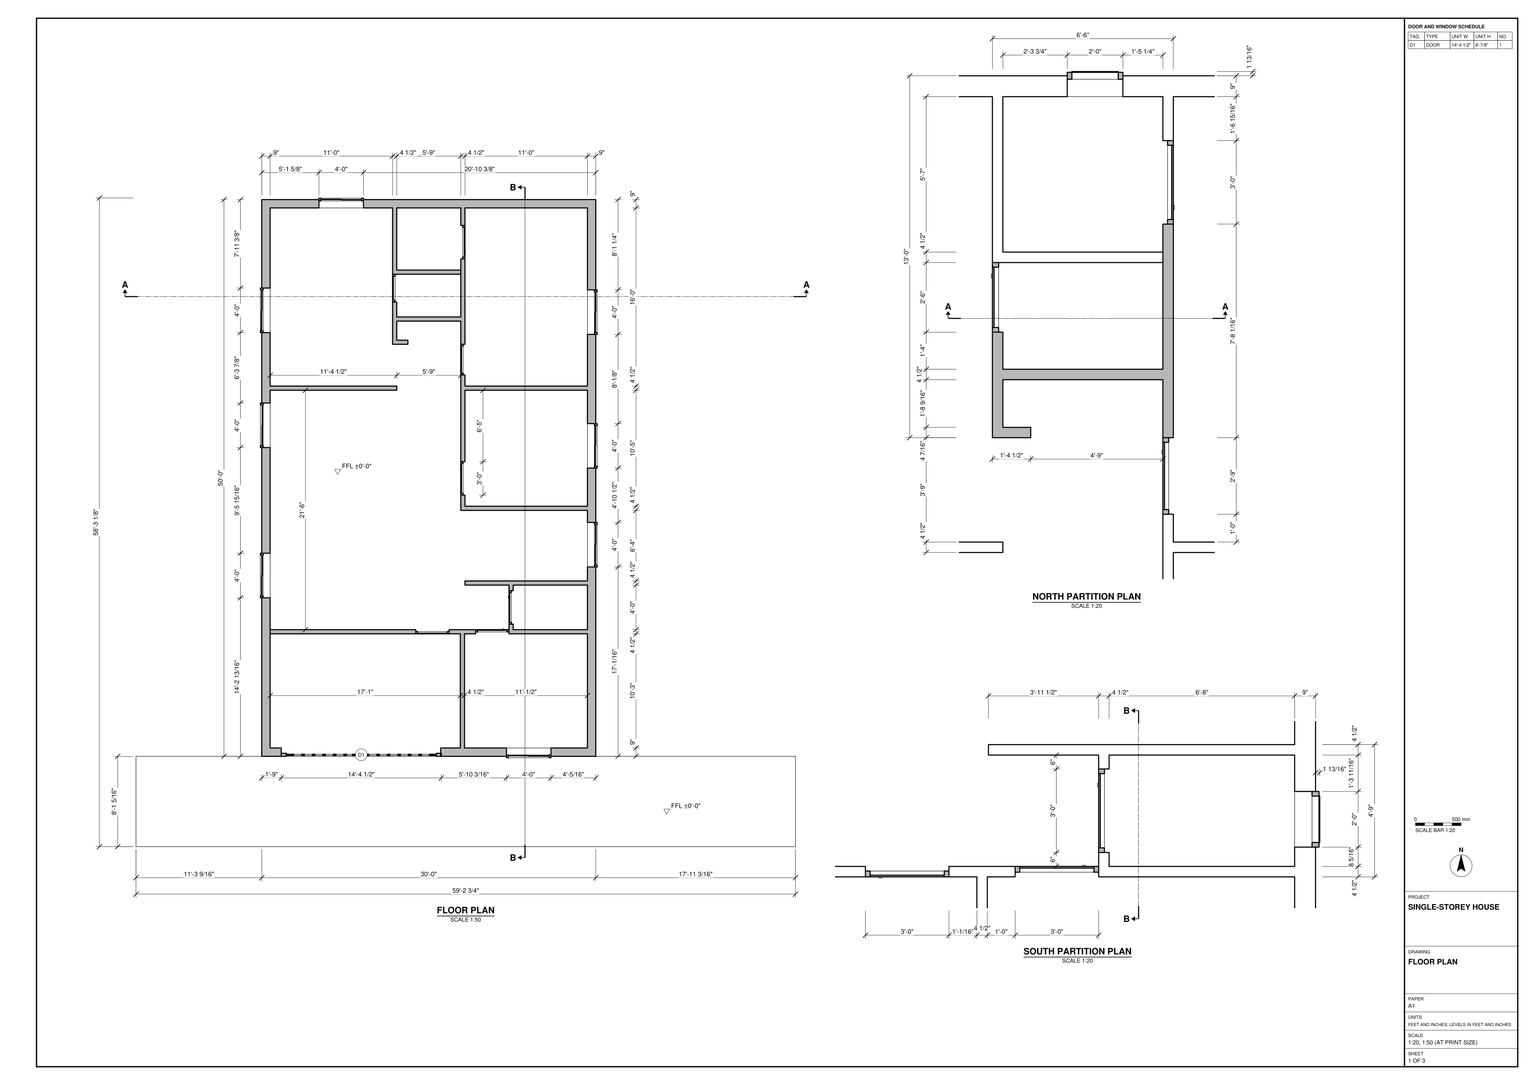
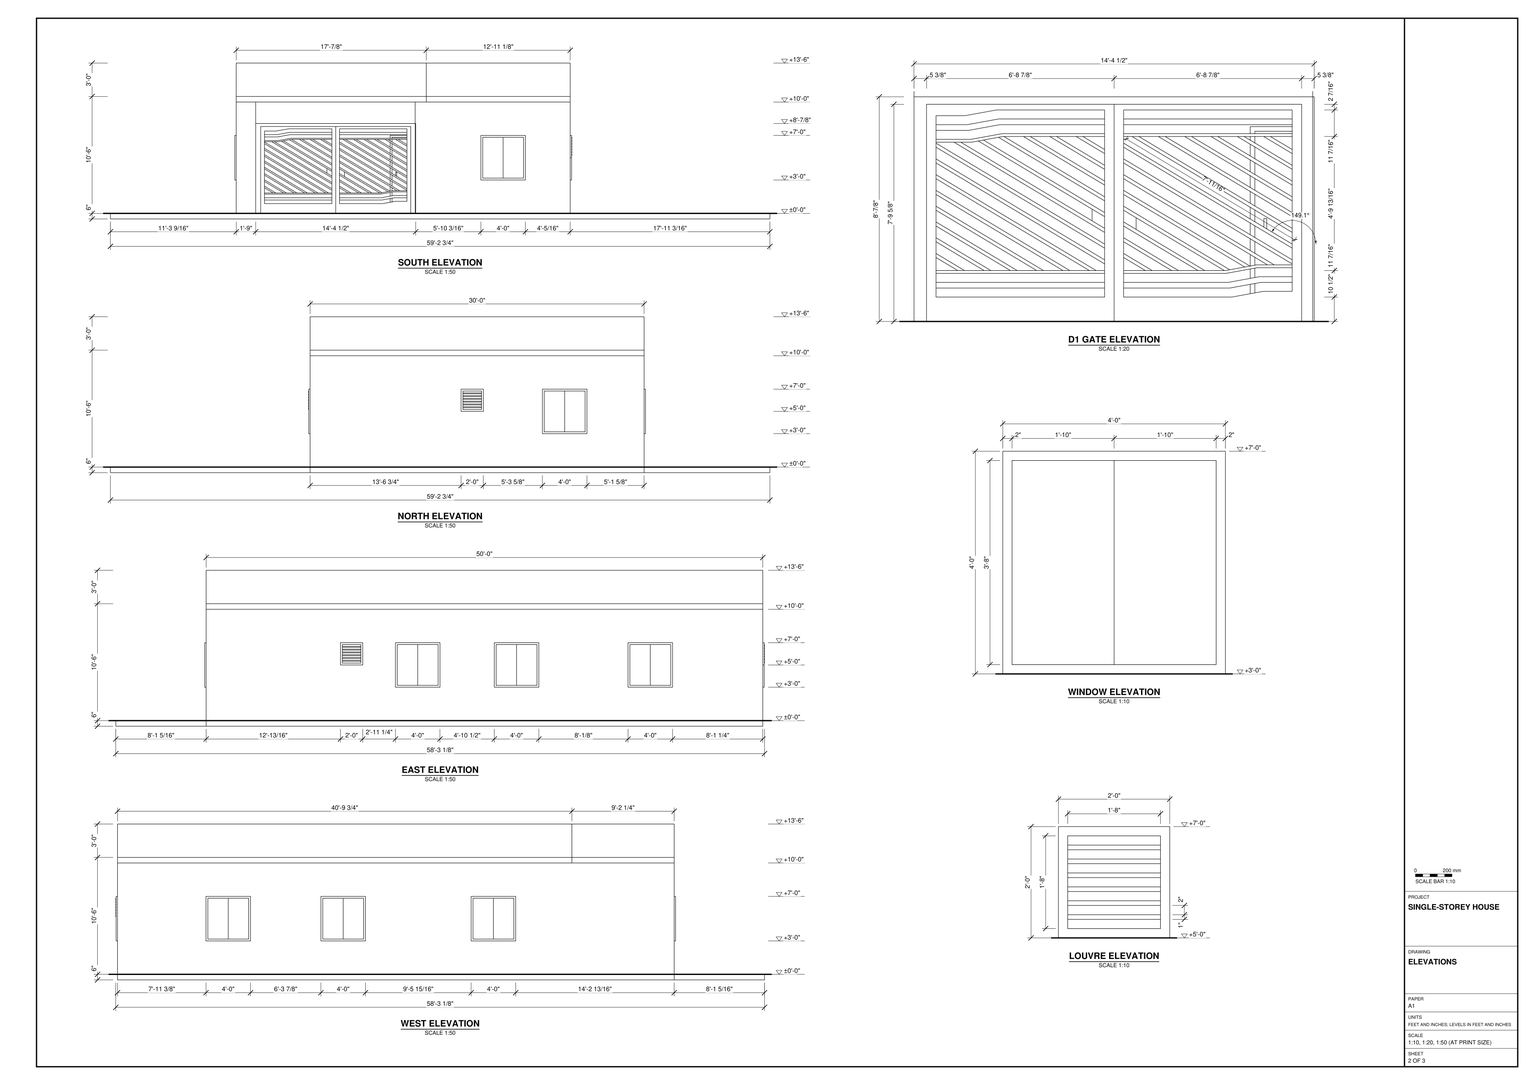
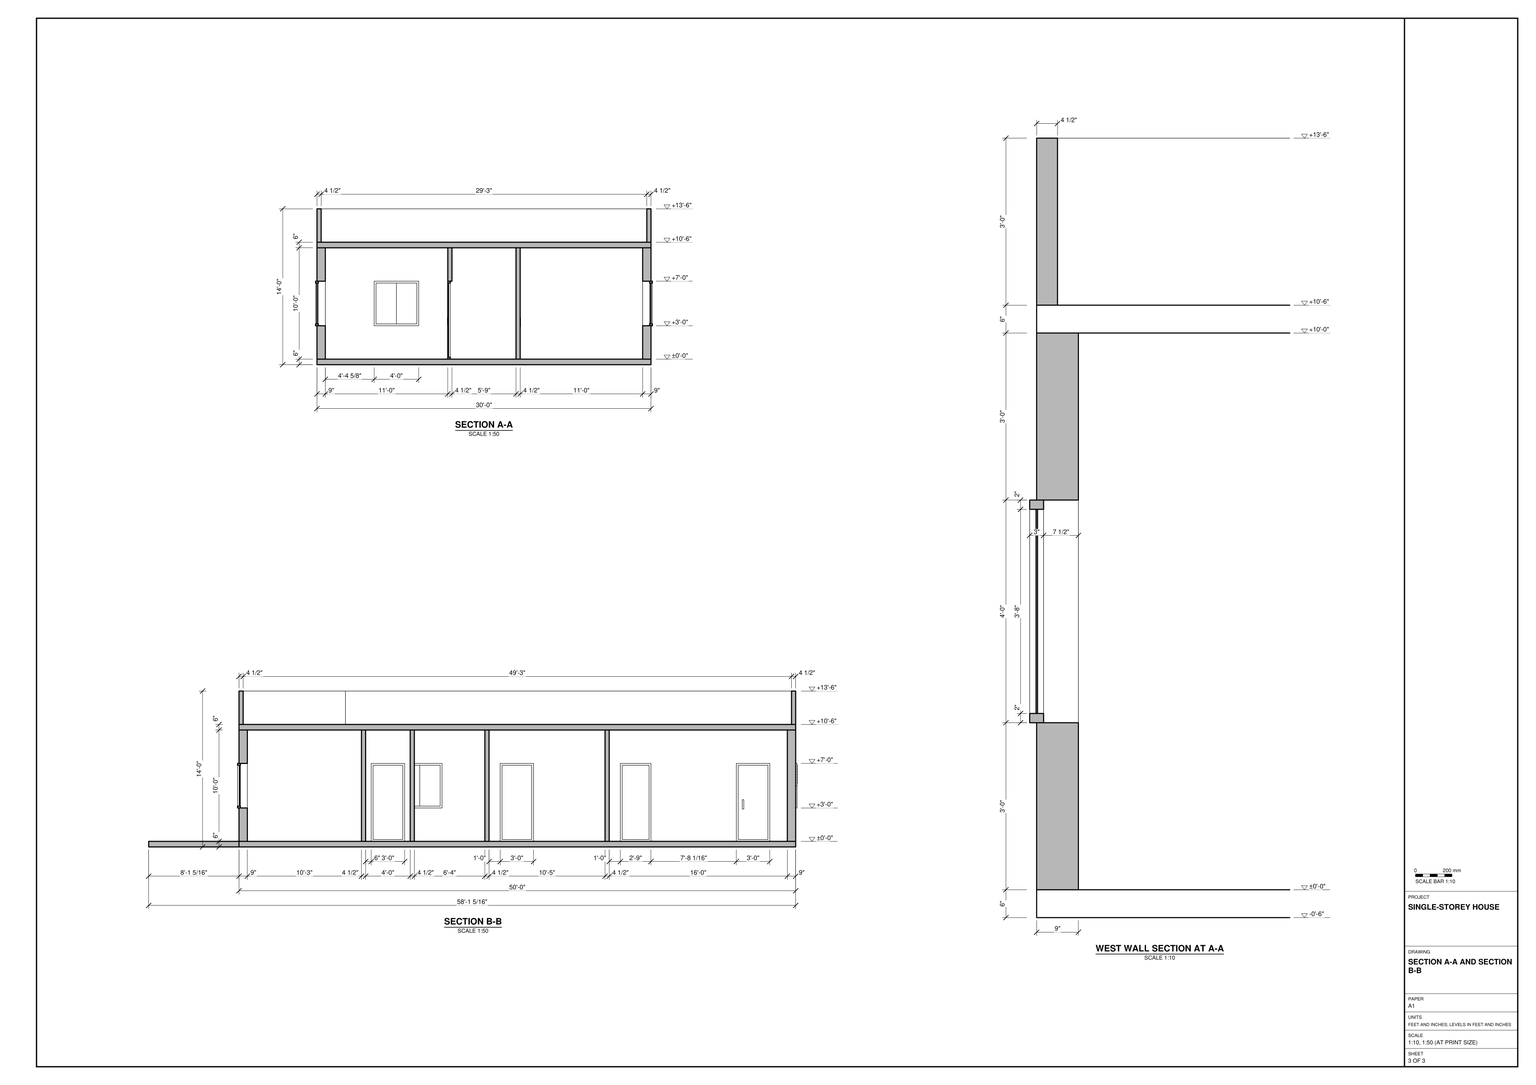
Build the single-storey house in SketchUp from task_files/diagram_01.pdf. Work in feet and inches and set the finished floor level to ±0'-0". The enclosed house measures 30'-0" east to west by 50'-0" north to south. Include the front slab that projects south of the house and extends beyond both side walls. The overall model extents, including this slab, are 59'-2 3/4" along X, 58'-3 1/8" along Y and 14'-0" along Z.

Lay out the 9" exterior walls and 4 1/2" interior partitions from the floor plan. Use the enlarged north and south partition plans to place the short wall returns and doorways. Fit the wide, two-leaf gate in the south wall, with its diagonal bars and the separate window to its right when viewed from outside. Follow the elevations for the positions of the divided windows and the smaller louvred openings. Use the sections to set the ground slab, flat roof slab and perimeter parapet at their drawn thicknesses and heights.

Keep walls, slabs and roof separately grouped or componentised. Keep each furniture or joinery piece separate where shown, and use components for repeated parts such as the window units. Any decor or loose items may be suitable library components. Save one SketchUp model as output_files/single_storey_house_with_its_front_gate_and_parapet.skp.

# SketchUp Ruby script. Lengths in inches.
U = 1.inch
M = Sketchup.active_model
def pt(a) = Geom::Point3d.new(a.map { |v| v * U })
def face(e, loops, mat)
  f = e.add_face(loops[0].map { |a| pt(a) })
  loops[1..].each { |l| e.add_face(l.map { |a| pt(a) }).erase! }
  f.material = f.back_material = mat if mat
  f
end
# faces: each face lists its corners as indices into pts; further lists are holes
def faces(e, pts, list, mat = nil) = list.each { |f| face(e, (f[0].is_a?(Array) ? f : [f]).map { |l| l.map { |i| pts[i] } }, mat) }
# xy, xz, yz: faces in a plane at the given z, y or x. An outline is a flat list of corners, or four numbers for a rectangle; further outlines are holes
def ring(l) = l.size == 4 ? [[l[0], l[1]], [l[2], l[1]], [l[2], l[3]], [l[0], l[3]]] : l.each_slice(2).to_a
def flat(e, list, mat, &to3) = list.each { |f| face(e, (f[0].is_a?(Array) ? f : [f]).map { |l| ring(l).map { |u, v| to3.(u, v) } }, mat) }
def xy(e, z, list, mat = nil) = flat(e, list, mat) { |x, y| [x, y, z] }
def xz(e, y, list, mat = nil) = flat(e, list, mat) { |x, z| [x, y, z] }
def yz(e, x, list, mat = nil) = flat(e, list, mat) { |y, z| [x, y, z] }
def lines(e, pts, list) = list.each { |a, b| e.add_line(pt(pts[a]), pt(pts[b])) }
# prism: a flat outline (further loops are holes) pulled along v
def prism(e, loops, v, mat = nil)
  f = face(e, loops, mat); d = Geom::Vector3d.new(v.map { |x| x * U })
  f.pushpull(f.normal.samedirection?(d) ? d.length : -d.length)
end
def box(e, o, s, mat = nil) = prism(e, [[o, [o[0] + s[0], o[1], o[2]], [o[0] + s[0], o[1] + s[1], o[2]], [o[0], o[1] + s[1], o[2]]]], [0, 0, s[2]], mat)
def at(x, y, z, deg = 0) = Geom::Transformation.translation(pt([x, y, z])) * Geom::Transformation.rotation(ORIGIN, Z_AXIS, deg.degrees)
def axes(o, x, y, z) = Geom::Transformation.new([*x, 0, *y, 0, *z, 0, *pt(o).to_a, 1])
def part(name) = M.definitions.add(name)
# library, detail: a bought-in or finely detailed component or shape, given as its bounding box
def library(name, o, s) = part(name).tap { |d| box(d.entities, o, s) }
def detail(e, o, s) = box(e.add_group.entities, o, s)
def put(e, d, t, mat = nil) = e.add_instance(d, t).tap { |i| i.material = mat if mat }
def group(e, t, mat = nil) = e.add_group.tap { |g| g.transformation = t; g.material = mat if mat }.entities
root = M.entities
M.materials.add("Flooring Laminate C Narrow 250cm").color = [165, 129, 108]
M.materials.add("Glass Smoked Distorted 001").color = [38, 38, 38]
M.materials["Glass Smoked Distorted 001"].alpha = 0.1
M.materials.add("Granite Black Pearl 150cm").color = [48, 48, 48]
M.materials.add("Iron Blurry").color = [53, 53, 53]
M.materials.add("Paper A 20cm").color = [184, 151, 117]
M.materials.add("Plaster Black Smooth 300cm").color = [38, 38, 38]
M.materials.add("Plaster Poised Taupe Smooth 300cm").color = [140, 135, 132]
M.materials.add("Plaster White Smooth 300cm").color = [216, 216, 216]
c1 = library("gate 109k\#1",[0,0.71,0],[103.31,3.23,96.85])
c2 = library("Dome Light",[-12,-12,0],[24,24,12])
c3 = part("Group\#3")
box(c3.entities,[0,0,0],[22,0.31,44])
c4 = part("Group\#5")
box(c4.entities,[0,0,0],[0.31,20,2])
c5 = part("Group\#7")
box(c5.entities,[-0.31,0,0],[0.31,22,44])
c6 = part("Group\#9")
box(c6.entities,[-0.31,0,0],[0.31,22,44])
c7 = part("Group\#11")
box(c7.entities,[-0.31,0,0],[0.31,22,44])
c8 = part("Group\#13")
box(c8.entities,[0,0,0],[20,0.31,2])
c9 = part("Group\#15")
box(c9.entities,[0,-0.31,0],[22,0.31,44])
c10 = part("Group\#17")
box(c10.entities,[0,0,0],[0.31,22,44])
c11 = part("Group\#19")
box(c11.entities,[-0.31,0,0],[0.31,22,44])
c12 = part("Group\#21")
box(c12.entities,[-0.31,0,0],[0.31,22,44])
put(root,c1,axes([156.5625,96.625,0],[1.67,0,0],[0,1,0],[0,0,1]))
put(root,c2,at(121.89,55.36,34.79))
g1 = group(root,at(135.5625,97.33,0))
xy(g1,0,[[21,0,192.88,0,192.88,9,214,9,214,132,201.9375,132,201.9375,136.5,230.5,136.5,230.5,132,218.5,132,218.5,9,351,9,351,132,266.5,132,266.5,142.5,271,142.5,271,136.5,351,136.5,351,184.5,271,184.5,271,178.5,266.5,178.5,266.5,184.5,219,184.5,219,189,351,189,351,265,214.5,265,214.5,281.5,219,281.5,219,269.5,351,269.5,351,394.5,219,394.5,219,317.5,214.5,317.5,214.5,411,219,411,219,399,351,399,351,591,219,591,219,572.0625,214.5,572.0625,214.5,591,145.5,591,145.5,524,214.5,524,214.5,536.0625,219,536.0625,219,444,214.5,444,214.5,469,145.5,469,145.5,448.4375,157.5,448.4375,157.5,444,141,444,141,489.5,145.5,489.5,145.5,473.5,214.5,473.5,214.5,519.5,141,519.5,141,591,9,591,9,399,145.5,399,145.5,394.5,9,394.5,9,136.5,165.9375,136.5,165.9375,132,9,132,9,9,21,9]],"Granite Black Pearl 150cm")
xy(g1,36,[[263.7,0,311.7,9],[0,170.83,9,218.83],[351,204.0625,360,252.0625],[351,310.59,360,358.59],[0,332.75,9,380.75],
  [351,454.72,360,502.72],[0,456.625,9,504.625],[61.62,591,109.62,600]])
xy(g1,60,[[351,144.8125,360,168.8125],[173.25,591,197.25,600]])
xy(g1,84,[[263.7,0,311.7,9],[165.9375,132,201.9375,136.5],[230.5,132,266.5,136.5],[266.5,142.5,271,178.5],[351,144.8125,360,168.8125],
  [0,170.83,9,218.83],[351,204.0625,360,252.0625],[214.5,281.5,219,317.5],[351,310.59,360,358.59],[0,332.75,9,380.75],
  [141,399,145.5,444],[214.5,411,214.5,444,157.5,444,157.5,448.4375,214.5,448.4375,214.5,444,219,444,219,411],[351,454.72,360,502.72],[0,456.625,9,504.625],[141,489.5,145.5,519.5],
  [214.5,536.0625,219,572.0625],[61.62,591,109.62,600],[173.25,591,197.25,600]])
xy(g1,120,[[[0,0,21,0,21,9,9,9,9,394.5,145.5,394.5,145.5,444,214.5,444,214.5,265,351,265,351,189,219,189,219,184.5,266.5,184.5,266.5,136.5,9,136.5,9,132,214,132,214,9,192.88,9,192.88,0,360,0,360,600,0,600],[219,399,351,591],[9,399,141,591],[219,269.5,351,394.5],[218.5,9,351,132],[145.5,473.5,145.5,519.5,214.5,519.5,214.5,524,145.5,524,145.5,591,214.5,591,214.5,473.5],[271,136.5,351,184.5],[145.5,448.4375,214.5,469]]])
xz(g1,0,[[0,0,21,120],[[192.88,0,360,120],[263.7,36,311.7,84]]],"Plaster Poised Taupe Smooth 300cm")
xz(g1,9,[[9,0,21,120],[192.88,0,214,120]])
xz(g1,9,[[[218.5,0,351,120],[263.7,36,311.7,84]]],"Paper A 20cm")
xz(g1,132,[[9,0,165.9375,0,165.9375,84,201.9375,84,201.9375,0,214,0,214,120,9,120],[218.5,0,230.5,0,230.5,84,266.5,84,266.5,0,351,0,351,120,218.5,120]],"Paper A 20cm")
xz(g1,136.5,[[9,0,9,120,266.5,120,266.5,84,230.5,84,230.5,0,201.9375,0,201.9375,84,165.9375,84,165.9375,0],[271,0,351,120]],"Paper A 20cm")
xz(g1,142.5,[[266.5,0,271,84]])
xz(g1,144.8125,[[351,60,360,84]])
xz(g1,168.8125,[[351,60,360,84]])
xz(g1,170.83,[[0,36,9,84]])
xz(g1,178.5,[[266.5,0,271,84]])
xz(g1,184.5,[[219,0,266.5,120],[271,0,351,120]],"Paper A 20cm")
xz(g1,189,[[219,0,351,120]],"Paper A 20cm")
xz(g1,204.0625,[[351,36,360,84]])
xz(g1,218.83,[[0,36,9,84]])
xz(g1,252.0625,[[351,36,360,84]])
xz(g1,265,[[214.5,0,351,120]],"Paper A 20cm")
xz(g1,269.5,[[219,0,351,120]],"Paper A 20cm")
xz(g1,281.5,[[214.5,0,219,84]])
xz(g1,310.59,[[351,36,360,84]])
xz(g1,317.5,[[214.5,0,219,84]])
xz(g1,332.75,[[0,36,9,84]])
xz(g1,358.59,[[351,36,360,84]])
xz(g1,380.75,[[0,36,9,84]])
xz(g1,394.5,[[9,0,145.5,120],[219,0,351,120]],"Paper A 20cm")
xz(g1,399,[[9,0,9,120,141,120,141,84,145.5,84,145.5,0],[219,0,351,120]],"Paper A 20cm")
xz(g1,411,[[214.5,0,219,84]])
xz(g1,444,[[214.5,0,219,84]])
xz(g1,444,[[141,0,157.5,0,157.5,84,214.5,84,214.5,120,145.5,120,145.5,84,141,84]],"Paper A 20cm")
xz(g1,448.4375,[[145.5,0,145.5,120,214.5,120,214.5,84,157.5,84,157.5,0]],"Paper A 20cm")
xz(g1,454.72,[[351,36,360,84]])
xz(g1,456.625,[[0,36,9,84]])
xz(g1,469,[[145.5,0,214.5,120]],"Paper A 20cm")
xz(g1,473.5,[[145.5,0,214.5,120]],"Paper A 20cm")
xz(g1,489.5,[[141,0,145.5,84]])
xz(g1,502.72,[[351,36,360,84]])
xz(g1,504.625,[[0,36,9,84]])
xz(g1,519.5,[[141,0,214.5,0,214.5,120,145.5,120,145.5,84,141,84]],"Paper A 20cm")
xz(g1,524,[[145.5,0,214.5,120]],"Paper A 20cm")
xz(g1,536.0625,[[214.5,0,219,84]])
xz(g1,572.0625,[[214.5,0,219,84]])
xz(g1,591,[[[9,0,141,120],[61.62,36,109.62,84]],[[145.5,0,214.5,120],[173.25,60,197.25,84]],[219,0,351,120]],"Paper A 20cm")
xz(g1,600,[[[0,0,360,120],[61.62,36,109.62,84],[173.25,60,197.25,84]]],"Plaster White Smooth 300cm")
yz(g1,0,[[[0,0,600,120],[456.625,36,504.625,84],[332.75,36,380.75,84],[170.83,36,218.83,84]]],"Plaster White Smooth 300cm")
yz(g1,9,[[132,0,136.5,120]])
yz(g1,9,[[9,0,132,120],[[136.5,0,394.5,120],[332.75,36,380.75,84],[170.83,36,218.83,84]],[[399,0,591,120],[456.625,36,504.625,84]]],"Paper A 20cm")
yz(g1,21,[[0,0,9,120]])
yz(g1,61.62,[[591,36,600,84]])
yz(g1,109.62,[[591,36,600,84]])
yz(g1,141,[[444,0,444,84,399,84,399,120,591,120,591,0,519.5,0,519.5,84,489.5,84,489.5,0]],"Paper A 20cm")
yz(g1,145.5,[[394.5,0,399,0,399,84,444,84,444,120,394.5,120],[448.4375,0,469,120],[473.5,0,489.5,0,489.5,84,519.5,84,519.5,120,473.5,120],[524,0,591,120]],"Paper A 20cm")
yz(g1,157.5,[[444,0,448.4375,84]])
yz(g1,165.9375,[[132,0,136.5,84]])
yz(g1,173.25,[[591,60,600,84]])
yz(g1,192.88,[[0,0,9,120]])
yz(g1,197.25,[[591,60,600,84]])
yz(g1,201.9375,[[132,0,136.5,84]])
yz(g1,214,[[9,0,132,120]],"Paper A 20cm")
yz(g1,214.5,[[519.5,0,524,120]])
yz(g1,214.5,[[265,0,265,120,444,120,444,84,411,84,411,0,317.5,0,317.5,84,281.5,84,281.5,0],[444,0,444,84,448.4375,84,448.4375,120,469,120,469,0],[473.5,0,519.5,120],[524,0,524,120,591,120,591,0,572.0625,0,572.0625,84,536.0625,84,536.0625,0]],"Paper A 20cm")
yz(g1,218.5,[[9,0,132,120]],"Paper A 20cm")
yz(g1,219,[[184.5,0,189,120]])
yz(g1,219,[[269.5,0,281.5,0,281.5,84,317.5,84,317.5,0,394.5,0,394.5,120,269.5,120],[399,0,411,0,411,84,444,84,444,0,536.0625,0,536.0625,84,572.0625,84,572.0625,0,591,0,591,120,399,120]],"Paper A 20cm")
yz(g1,230.5,[[132,0,136.5,84]])
yz(g1,263.7,[[0,36,9,84]])
yz(g1,266.5,[[132,0,132,84,136.5,84,136.5,120,184.5,120,184.5,0,178.5,0,178.5,84,142.5,84,142.5,0]],"Paper A 20cm")
yz(g1,271,[[136.5,0,142.5,0,142.5,84,178.5,84,178.5,0,184.5,0,184.5,120,136.5,120]],"Paper A 20cm")
yz(g1,311.7,[[0,36,9,84]])
yz(g1,351,[[9,0,132,120],[[136.5,0,184.5,120],[144.8125,60,168.8125,84]],[[189,0,265,120],[204.0625,36,252.0625,84]],[[269.5,0,394.5,120],[310.59,36,358.59,84]],[[399,0,591,120],[454.72,36,502.72,84]]],"Paper A 20cm")
yz(g1,360,[[[0,0,600,120],[204.0625,36,252.0625,84],[310.59,36,358.59,84],[454.72,36,502.72,84],[144.8125,60,168.8125,84]]],"Plaster White Smooth 300cm")
g2 = group(g1,at(263.7,0,36))
prism(g2,[[[0,-1.5,0],[48,-1.5,0],[48,-1.5,48],[0,-1.5,48]],[[2,-1.5,46],[46,-1.5,46],[46,-1.5,2],[2,-1.5,2]]],[0,3,0],"Iron Blurry")
put(g2,c3,at(2,0.5,2),"Glass Smoked Distorted 001")
put(g2,c3,at(24,0.19,2),"Glass Smoked Distorted 001")
g3 = group(g1,at(360,144.8125,60))
prism(g3,[[[1.5,0,0],[1.5,24,0],[1.5,24,24],[1.5,0,24]],[[1.5,2,2],[1.5,2,22],[1.5,22,22],[1.5,22,2]]],[-3,0,0],"Iron Blurry")
put(g3,c4,at(1.5,2,20),"Glass Smoked Distorted 001")
put(g3,c4,at(1.5,2,17),"Glass Smoked Distorted 001")
put(g3,c4,at(1.5,2,14),"Glass Smoked Distorted 001")
put(g3,c4,at(1.5,2,11),"Glass Smoked Distorted 001")
put(g3,c4,at(1.5,2,8),"Glass Smoked Distorted 001")
put(g3,c4,at(1.5,2,5),"Glass Smoked Distorted 001")
put(g3,c4,at(1.5,2,2),"Glass Smoked Distorted 001")
g4 = group(g1,at(360,204.0625,36))
prism(g4,[[[1.5,48,0],[1.5,48,48],[1.5,0,48],[1.5,0,0]],[[1.5,2,46],[1.5,46,46],[1.5,46,2],[1.5,2,2]]],[-3,0,0],"Iron Blurry")
put(g4,c5,at(-0.25,2,2),"Glass Smoked Distorted 001")
put(g4,c5,at(0.06,24,2),"Glass Smoked Distorted 001")
g5 = group(g1,at(360,310.59,36))
prism(g5,[[[1.5,0,0],[1.5,48,0],[1.5,48,48],[1.5,0,48]],[[1.5,46,46],[1.5,46,2],[1.5,2,2],[1.5,2,46]]],[-3,0,0],"Iron Blurry")
put(g5,c6,at(-0.5,2,2),"Glass Smoked Distorted 001")
put(g5,c6,at(-0.19,24,2),"Glass Smoked Distorted 001")
g6 = group(g1,at(360,454.72,36))
prism(g6,[[[1.5,0,0],[1.5,48,0],[1.5,48,48],[1.5,0,48]],[[1.5,46,2],[1.5,2,2],[1.5,2,46],[1.5,46,46]]],[-3,0,0],"Iron Blurry")
put(g6,c7,at(-0.3125,2,2),"Glass Smoked Distorted 001")
put(g6,c7,at(0,24,2),"Glass Smoked Distorted 001")
g7 = group(g1,at(173.25,600,60))
prism(g7,[[[24,1.5,0],[0,1.5,0],[0,1.5,24],[24,1.5,24]],[[2,1.5,22],[2,1.5,2],[22,1.5,2],[22,1.5,22]]],[0,-3,0],"Iron Blurry")
put(g7,c8,at(2,1.5,20),"Glass Smoked Distorted 001")
put(g7,c8,at(2,1.5,17),"Glass Smoked Distorted 001")
put(g7,c8,at(2,1.5,14),"Glass Smoked Distorted 001")
put(g7,c8,at(2,1.5,11),"Glass Smoked Distorted 001")
put(g7,c8,at(2,1.5,8),"Glass Smoked Distorted 001")
put(g7,c8,at(2,1.5,5),"Glass Smoked Distorted 001")
put(g7,c8,at(2,1.5,2),"Glass Smoked Distorted 001")
g8 = group(g1,at(61.62,600,36))
prism(g8,[[[0,1.5,0],[0,1.5,48],[48,1.5,48],[48,1.5,0]],[[2,1.5,2],[46,1.5,2],[46,1.5,46],[2,1.5,46]]],[0,-3,0],"Iron Blurry")
put(g8,c9,at(24,0,2),"Glass Smoked Distorted 001")
put(g8,c9,at(2,0.3125,2),"Glass Smoked Distorted 001")
g9 = group(g1,at(0,456.625,36))
prism(g9,[[[-1.5,48,0],[-1.5,0,0],[-1.5,0,48],[-1.5,48,48]],[[-1.5,2,2],[-1.5,46,2],[-1.5,46,46],[-1.5,2,46]]],[3,0,0],"Iron Blurry")
put(g9,c10,at(-0.125,24,2),"Glass Smoked Distorted 001")
put(g9,c10,at(-0.44,2,2),"Glass Smoked Distorted 001")
g10 = group(g1,at(0,332.75,36))
prism(g10,[[[-1.5,48,0],[-1.5,0,0],[-1.5,0,48],[-1.5,48,48]],[[-1.5,46,2],[-1.5,46,46],[-1.5,2,46],[-1.5,2,2]]],[3,0,0],"Iron Blurry")
put(g10,c11,at(0.8125,24,2),"Glass Smoked Distorted 001")
put(g10,c11,at(0.5,2,2),"Glass Smoked Distorted 001")
g11 = group(g1,at(0,170.83,36))
prism(g11,[[[-1.5,48,0],[-1.5,0,0],[-1.5,0,48],[-1.5,48,48]],[[-1.5,46,46],[-1.5,2,46],[-1.5,2,2],[-1.5,46,2]]],[3,0,0],"Iron Blurry")
put(g11,c12,at(0.4375,24,2),"Glass Smoked Distorted 001")
put(g11,c12,at(0.12,2,2),"Glass Smoked Distorted 001")
g12 = group(g1,at(165.9375,132,0))
xy(g12,0,[[0,0,36,2.5]])
xy(g12,2,[[2,0,34,2.5]])
xy(g12,82,[[2,0,34,2.5]])
xy(g12,84,[[0,0,36,2.5]])
xz(g12,0,[[[0,0,36,84],[2,2,34,82]]],"Iron Blurry")
xz(g12,2.5,[[[0,0,36,84],[2,2,34,82]]])
yz(g12,0,[[0,0,2.5,84]])
yz(g12,2,[[0,2,2.5,82]])
yz(g12,34,[[0,2,2.5,82]])
yz(g12,36,[[0,0,2.5,84]])
g13 = group(g12,at(2,0,2))
box(g13,[0,0,0],[32,0.71,80],"Flooring Laminate C Narrow 250cm")
g14 = group(g13,at(3.88,0,37.3125),"Iron Blurry")
box(g14,[0,-0.5,0],[1.25,0.5,5.0625])
g15 = group(g1,at(141,489.5,0))
prism(g15,[[[0,0,0],[0,0,84],[0,30,84],[0,30,0]],[[0,28,2],[0,28,82],[0,2,82],[0,2,2]]],[2.6875,0,0],"Iron Blurry")
g16 = group(g15,at(0,2,2),"Flooring Laminate C Narrow 250cm")
box(g16,[0,0,0],[0.71,26,80],"Flooring Laminate C Narrow 250cm")
g17 = group(g16,at(0,23.02,35.27),"Iron Blurry")
box(g17,[-0.5,-1.72,0],[0.5,1.72,8.06],"Iron Blurry")
g18 = group(g1,at(214.5,411,0))
prism(g18,[[[0,0,0],[0,0,84],[0,33,84],[0,33,0]],[[0,31,82],[0,2,82],[0,2,2],[0,31,2]]],[2.5,0,0],"Iron Blurry")
g19 = group(g18,at(0,2,2))
xy(g19,0,[[0,0,0.71,29]])
xy(g19,80,[[0,0,0.71,29]])
xz(g19,0,[[0,0,0.71,80]])
xz(g19,29,[[0,0,0.71,80]])
yz(g19,0,[[0,0,29,80]],"Flooring Laminate C Narrow 250cm")
yz(g19,0.71,[[0,0,29,80]],"Flooring Laminate C Narrow 250cm")
g20 = group(g19,at(0,25.625,34.73),"Iron Blurry")
box(g20,[-0.5,-1.5625,0],[0.5,1.5625,7.0625])
g21 = group(g1,at(214.5,281.5,0))
prism(g21,[[[0,0,0],[0,0,84],[0,36,84],[0,36,0]],[[0,34,2],[0,34,82],[0,2,82],[0,2,2]]],[2.5,0,0],"Iron Blurry")
g22 = group(g21,at(0,2,2),"Flooring Laminate C Narrow 250cm")
box(g22,[0,0,0],[0.71,32,80],"Flooring Laminate C Narrow 250cm")
g23 = group(g22,at(0,26.78,37.39),"Iron Blurry")
box(g23,[-0.5,-1.75,0],[0.5,1.75,5.87],"Iron Blurry")
g24 = group(g1,at(219,536.0625,0))
prism(g24,[[[0,36,0],[0,36,84],[0,0,84],[0,0,0]],[[0,2,82],[0,34,82],[0,34,2],[0,2,2]]],[-2.5,0,0],"Iron Blurry")
g25 = group(g24,at(0,2,2))
xy(g25,0,[[-0.71,0,0,32]])
xy(g25,80,[[-0.71,0,0,32]])
xz(g25,0,[[-0.71,0,0,80]])
xz(g25,32,[[-0.71,0,0,80]])
yz(g25,-0.71,[[0,0,32,80]],"Flooring Laminate C Narrow 250cm")
yz(g25,0,[[0,0,32,80]],"Flooring Laminate C Narrow 250cm")
g26 = group(g25,at(0,4.38,32.8125),"Iron Blurry")
box(g26,[0,0,0],[0.5,1.625,10.125],"Iron Blurry")
g27 = group(g1,at(266.5,142.5,0))
xy(g27,0,[[0,0,2.5,36]])
xy(g27,2,[[0,2,2.5,34]])
xy(g27,82,[[0,2,2.5,34]])
xy(g27,84,[[0,0,2.5,36]])
xz(g27,0,[[0,0,2.5,84]])
xz(g27,2,[[0,2,2.5,82]])
xz(g27,34,[[0,2,2.5,82]])
xz(g27,36,[[0,0,2.5,84]])
yz(g27,0,[[[0,0,36,84],[2,2,34,82]]],"Iron Blurry")
yz(g27,2.5,[[[0,0,36,84],[2,2,34,82]]])
g28 = group(g27,at(0,2,2))
box(g28,[0,0,0],[0.71,32,80],"Flooring Laminate C Narrow 250cm")
g29 = group(g28,at(0,27.88,36.06),"Iron Blurry")
box(g29,[-0.5,-1.625,0],[0.5,1.625,9.5625],"Iron Blurry")
g30 = group(g1,at(230.5,136.5,0))
xy(g30,0,[[0,-2.5,36,0]])
xy(g30,2,[[2,-2.5,34,0]])
xy(g30,82,[[2,-2.5,34,0]])
xy(g30,84,[[0,-2.5,36,0]])
xz(g30,-2.5,[[[0,0,36,84],[2,2,34,82]]])
xz(g30,0,[[[0,0,36,84],[2,2,34,82]]],"Iron Blurry")
yz(g30,0,[[-2.5,0,0,84]])
yz(g30,2,[[-2.5,2,0,82]])
yz(g30,34,[[-2.5,2,0,82]])
yz(g30,36,[[-2.5,0,0,84]])
g31 = group(g30,at(2,0,2),"Flooring Laminate C Narrow 250cm")
box(g31,[0,-0.71,0],[32,0.71,80],"Flooring Laminate C Narrow 250cm")
g32 = group(g31,at(28.3125,0,39.4375),"Iron Blurry")
box(g32,[-1.25,0,0],[1.25,0.5,8.375],"Iron Blurry")
g33 = group(root,at(135.5625,97.33,120),"Plaster White Smooth 300cm")
box(g33,[0,0,-126],[360,600,6],"Granite Black Pearl 150cm")
xy(g33,0,[[204.88,0,204.88,110.25,0,110.25,0,600,360,600,360,0]],"Granite Black Pearl 150cm")
xy(g33,6,[[204.88,0,360,0,360,600,0,600,0,110.25,204.88,110.25]],"Plaster White Smooth 300cm")
xz(g33,0,[[204.88,0,360,6]],"Granite Black Pearl 150cm")
xz(g33,110.25,[[0,0,204.88,6]],"Granite Black Pearl 150cm")
xz(g33,600,[[0,0,360,6]],"Granite Black Pearl 150cm")
yz(g33,0,[[110.25,0,600,6]],"Granite Black Pearl 150cm")
yz(g33,204.88,[[0,0,110.25,6]],"Granite Black Pearl 150cm")
yz(g33,360,[[0,0,600,6]],"Granite Black Pearl 150cm")
g34 = group(g33,at(0,0,6))
xy(g34,0,[[[204.88,0,204.88,110.25,0,110.25,0,600,360,600,360,0],[209.38,4.5,355.5,4.5,355.5,595.5,4.5,595.5,4.5,114.75,209.38,114.75]]],"Plaster White Smooth 300cm")
xy(g34,36,[[[204.88,0,360,0,360,600,0,600,0,110.25,204.88,110.25],[209.38,4.5,209.38,114.75,4.5,114.75,4.5,595.5,355.5,595.5,355.5,4.5]]],"Plaster White Smooth 300cm")
xz(g34,0,[[204.88,0,360,36]],"Plaster Poised Taupe Smooth 300cm")
xz(g34,4.5,[[209.38,0,355.5,36]],"Plaster White Smooth 300cm")
xz(g34,110.25,[[0,0,204.88,36]],"Plaster Poised Taupe Smooth 300cm")
xz(g34,114.75,[[4.5,0,209.38,36]],"Plaster White Smooth 300cm")
xz(g34,595.5,[[4.5,0,355.5,36]],"Plaster White Smooth 300cm")
xz(g34,600,[[0,0,360,36]],"Plaster White Smooth 300cm")
yz(g34,0,[[110.25,0,600,36]],"Plaster White Smooth 300cm")
yz(g34,4.5,[[114.75,0,595.5,36]],"Plaster White Smooth 300cm")
yz(g34,204.88,[[0,0,110.25,36]],"Plaster White Smooth 300cm")
yz(g34,209.38,[[4.5,0,114.75,36]],"Plaster White Smooth 300cm")
yz(g34,355.5,[[4.5,0,595.5,36]],"Plaster White Smooth 300cm")
yz(g34,360,[[0,0,600,36]],"Plaster White Smooth 300cm")
g35 = group(root,at(135.5625,0,-6),"Plaster Black Smooth 300cm")
box(g35,[-135.5625,0,0],[710.78,97.33,6])
